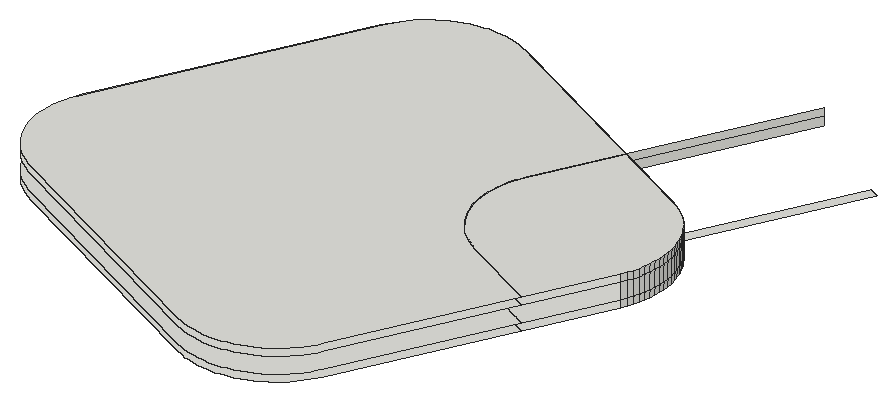
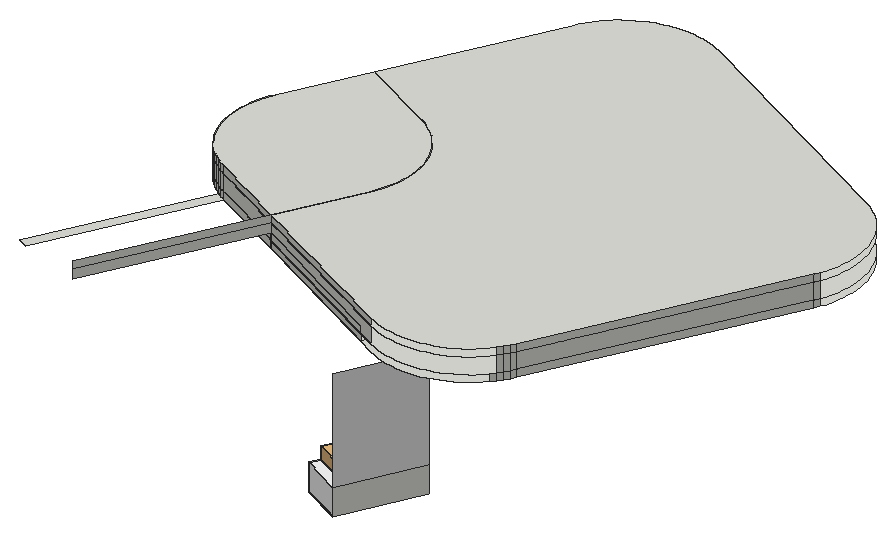
# SketchUp Ruby script. Lengths in inches.
U = 1.inch
M = Sketchup.active_model
def pt(a) = Geom::Point3d.new(a.map { |v| v * U })
def face(e, loops, mat)
  f = e.add_face(loops[0].map { |a| pt(a) })
  loops[1..].each { |l| e.add_face(l.map { |a| pt(a) }).erase! }
  f.material = f.back_material = mat if mat
  f
end
# faces: each face lists its corners as indices into pts; further lists are holes
def faces(e, pts, list, mat = nil) = list.each { |f| face(e, (f[0].is_a?(Array) ? f : [f]).map { |l| l.map { |i| pts[i] } }, mat) }
# xy, xz, yz: faces in a plane at the given z, y or x. An outline is a flat list of corners, or four numbers for a rectangle; further outlines are holes
def ring(l) = l.size == 4 ? [[l[0], l[1]], [l[2], l[1]], [l[2], l[3]], [l[0], l[3]]] : l.each_slice(2).to_a
def flat(e, list, mat, &to3) = list.each { |f| face(e, (f[0].is_a?(Array) ? f : [f]).map { |l| ring(l).map { |u, v| to3.(u, v) } }, mat) }
def xy(e, z, list, mat = nil) = flat(e, list, mat) { |x, y| [x, y, z] }
def xz(e, y, list, mat = nil) = flat(e, list, mat) { |x, z| [x, y, z] }
def yz(e, x, list, mat = nil) = flat(e, list, mat) { |y, z| [x, y, z] }
def lines(e, pts, list) = list.each { |a, b| e.add_line(pt(pts[a]), pt(pts[b])) }
# prism: a flat outline (further loops are holes) pulled along v
def prism(e, loops, v, mat = nil)
  f = face(e, loops, mat); d = Geom::Vector3d.new(v.map { |x| x * U })
  f.pushpull(f.normal.samedirection?(d) ? d.length : -d.length)
end
def box(e, o, s, mat = nil) = prism(e, [[o, [o[0] + s[0], o[1], o[2]], [o[0] + s[0], o[1] + s[1], o[2]], [o[0], o[1] + s[1], o[2]]]], [0, 0, s[2]], mat)
def at(x, y, z, deg = 0) = Geom::Transformation.translation(pt([x, y, z])) * Geom::Transformation.rotation(ORIGIN, Z_AXIS, deg.degrees)
def axes(o, x, y, z) = Geom::Transformation.new([*x, 0, *y, 0, *z, 0, *pt(o).to_a, 1])
def part(name) = M.definitions.add(name)
# library, detail: a bought-in or finely detailed component or shape, given as its bounding box
def library(name, o, s) = part(name).tap { |d| box(d.entities, o, s) }
def detail(e, o, s) = box(e.add_group.entities, o, s)
def put(e, d, t, mat = nil) = e.add_instance(d, t).tap { |i| i.material = mat if mat }
def group(e, t, mat = nil) = e.add_group.tap { |g| g.transformation = t; g.material = mat if mat }.entities
root = M.entities
M.materials.add("[Color_003]").color = [170, 170, 170]
M.materials.add("[Mirror 02]1").color = [230, 230, 230]
M.materials.add("[Plaster]").color = [253, 253, 253]
M.materials.add("[Translucent Glass Gray]14").color = [0, 0, 0]
M.materials["[Translucent Glass Gray]14"].alpha = 0.5
c1 = library("Pump dispenser pair",[-4.05,-18.11,-0.18],[3.15,7.24,8.23])
c2 = library("グループ\#54",[0,0,0],[6.36,0.94,9.53])
c3 = library("グループ\#83",[0,0.04,0],[11.77,11.73,3.9375])
c4 = part("Untitled1")
g1 = group(c4.entities,at(743.43,-253.09,0,-180))
xy(g1,0,[[0,0,554.6,297.75]],"[Plaster]")
xy(g1,29.71,[[41.91,287.06,269.97,291.99],[269.97,287.06,498.03,291.99]])
xy(g1,29.71,[[41.91,170.9375,498.03,287.06],[41.91,291.99,498.03,297.75]],"[Plaster]")
xy(g1,101.91,[[120.41,291.99,133.72,291.99,133.72,305.17,218.84,305.17,218.84,291.99,232.79,291.99,232.79,311.8,120.41,311.8],[305.71,291.99,312.55,291.99,312.55,305.42,407.55,305.42,407.55,291.99,418.08,291.99,418.08,312.8,305.71,312.8]],"[Translucent Glass Gray]14")
xy(g1,110.16,[[120.41,291.99,120.41,311.8,232.79,311.8,232.79,291.99,218.84,291.99,218.84,305.17,133.72,305.17,133.72,291.99],[305.71,291.99,305.71,312.8,418.08,312.8,418.08,291.99,407.55,291.99,407.55,305.42,312.55,305.42,312.55,291.99]],"[Translucent Glass Gray]14")
xy(g1,152.15,[[41.91,287.06,269.97,291.99],[269.97,287.06,498.03,291.99]])
xy(g1,152.15,[[41.91,170.9375,498.03,287.06],[41.91,291.99,498.03,297.75]],"[Plaster]")
xy(g1,175.18,[[0,0,554.6,297.75]],"[Plaster]")
xz(g1,0,[[0,0,554.6,175.18]])
xz(g1,0,[[0,175.18,554.6,861.94]],"[Mirror 02]1")
xz(g1,170.9375,[[41.91,29.71,498.03,152.15]],"[Plaster]")
xz(g1,287.06,[[41.91,29.71,269.97,152.15],[269.97,29.71,498.03,152.15]],"[Translucent Glass Gray]14")
xz(g1,291.99,[[[41.91,29.71,269.97,152.15],[218.84,101.91,232.79,110.16],[120.41,101.91,133.72,110.16]],[[269.97,29.71,498.03,152.15],[407.55,101.91,418.08,110.16],[305.71,101.91,312.55,110.16]]],"[Translucent Glass Gray]14")
xz(g1,297.75,[[[0,0,554.6,175.18],[41.91,29.71,498.03,152.15]]],"[Plaster]")
xz(g1,305.17,[[133.72,101.91,218.84,110.16]],"[Translucent Glass Gray]14")
xz(g1,305.42,[[312.55,101.91,407.55,110.16]],"[Translucent Glass Gray]14")
xz(g1,311.8,[[120.41,101.91,232.79,110.16]],"[Translucent Glass Gray]14")
xz(g1,312.8,[[305.71,101.91,418.08,110.16]],"[Translucent Glass Gray]14")
yz(g1,0,[[0,0,297.75,175.18]],"[Plaster]")
yz(g1,41.91,[[170.9375,29.71,287.06,152.15],[291.99,29.71,297.75,152.15]],"[Plaster]")
yz(g1,41.91,[[287.06,29.71,291.99,152.15]],"[Translucent Glass Gray]14")
yz(g1,120.41,[[291.99,101.91,311.8,110.16]],"[Translucent Glass Gray]14")
yz(g1,133.72,[[291.99,101.91,305.17,110.16]],"[Translucent Glass Gray]14")
yz(g1,218.84,[[291.99,101.91,305.17,110.16]],"[Translucent Glass Gray]14")
yz(g1,232.79,[[291.99,101.91,311.8,110.16]],"[Translucent Glass Gray]14")
yz(g1,269.97,[[287.06,29.71,291.99,152.15]],"[Translucent Glass Gray]14")
yz(g1,305.71,[[291.99,101.91,312.8,110.16]],"[Translucent Glass Gray]14")
yz(g1,312.55,[[291.99,101.91,305.42,110.16]],"[Translucent Glass Gray]14")
yz(g1,407.55,[[291.99,101.91,305.42,110.16]],"[Translucent Glass Gray]14")
yz(g1,418.08,[[291.99,101.91,312.8,110.16]],"[Translucent Glass Gray]14")
yz(g1,498.03,[[287.06,29.71,291.99,152.15]])
yz(g1,498.03,[[170.9375,29.71,287.06,152.15],[291.99,29.71,297.75,152.15]],"[Plaster]")
yz(g1,554.6,[[0,0,297.75,175.18]])
put(g1,c1,axes([334.9,116.79,177.8],[0,14.82,0],[-11.7078,0,0],[0,0,14.82]))
g2 = group(g1,at(68.38,2.16,176.47))
put(g2,c2,axes([147.62,131.72,21.69],[0,-20.70307,0],[29.98633,0,0],[0,0,20.70307]),"[Color_003]")
put(g2,c3,axes([-1.1,49.75,0],[0,20.70307,0],[29.98633,0,0],[0,0,20.70307]))
xy(root,412.84,[[[714.28,690.62,711.93,690.68,709.58,690.9,707.25,691.27,704.96,691.79,702.7,692.46,700.49,693.28,698.34,694.23,596.96,743.46,594.88,744.56,592.87,745.79,590.95,747.15,589.12,748.63,587.39,750.23,585.77,751.94,584.26,753.75,582.88,755.66,581.625,757.65,580.5,759.72,579.51,761.86,578.67,764.0625,577.97,766.3125,577.43,768.6,577.03,770.92,576.78,773.27,576.69,775.62,576.75,777.98,576.97,780.32,577.34,782.65,577.86,784.95,578.53,787.2,579.35,789.41,580.31,791.57,627.47,888.7,628.57,890.78,629.8,892.79,631.16,894.71,632.64,896.54,634.24,898.27,635.95,899.89,637.76,901.4,639.67,902.78,641.66,904.04,643.73,905.16,645.875,906.15,648.07,906.99,650.32,907.6875,652.61,908.24,654.9375,908.63,657.28,908.88,659.63,908.97,661.99,908.91,664.33,908.69,666.66,908.32,668.96,907.8,671.22,907.13,673.43,906.3125,675.58,905.36,682.44,902.02,666.72,869.64,671.22,867.45,686.94,899.84,744.57,871.86,728.84,839.47,727.88,837.32,727.06,835.11,726.39,832.85,725.875,830.56,725.5,828.23,725.29,825.88,725.23,823.53,725.32,821.17,725.5625,818.83,725.96,816.51,726.51,814.22,727.21,811.97,728.05,809.77,729.03,807.63,730.16,805.56,731.41,803.57,732.8,801.66,734.3,799.85,735.92,798.14,737.65,796.54,739.48,795.05,741.41,793.69,743.42,792.46,745.5,791.36,777.88,775.64,746.44,710.89,745.35,708.81,744.12,706.8,742.75,704.88,741.27,703.05,739.67,701.32,737.96,699.7,736.15,698.19,734.24,696.81,732.25,695.55,730.18,694.43,728.04,693.44,725.84,692.6,723.59,691.9,721.3,691.35,718.98,690.96,716.63,690.71],[616.59,773.95,663.75,871.08,659.85,872.97,612.69,775.84],[703.25,736.11,705.125,736.17,706.96,736.32,708.74,736.59,710.47,736.95,712.14,737.42,713.73,737.98,715.25,738.65,716.69,739.4,718.04,740.25,719.29,741.1875,720.45,742.2,721.5,743.3,722.43,744.47,723.26,745.72,723.97,747.02,729.79,759,728.6875,756.92,727.46,754.91,726.1,752.99,724.61,751.16,723.01,749.43,721.3,747.81,719.49,746.3,717.58,744.92,716.26,744.08,716.04,743.89,714.96,743.09,713.8,742.36,712.5625,741.7,711.25,741.13,709.88,740.65,708.44,740.24,706.96,739.93,706.02,739.79,704.64,739.46,702.32,739.06,699.98,738.82,697.62,738.73,695.27,738.79,692.92,739.01,690.59,739.375,688.3,739.9,686.04,740.57,683.83,741.38,681.68,742.34,685.99,740.25,687.85,739.4,689.74,738.64,691.66,737.98,693.59,737.42,695.54,736.95,697.49,736.59,699.43,736.32,701.35,736.17]],[616.59,773.95,612.69,775.84,659.85,872.97,663.75,871.08],[[777.88,775.64,745.5,791.36,743.42,792.46,741.41,793.69,739.48,795.05,737.65,796.54,735.92,798.14,734.3,799.85,732.8,801.66,731.41,803.57,730.16,805.56,729.03,807.63,728.05,809.77,727.21,811.97,726.51,814.22,725.96,816.51,725.5625,818.83,725.32,821.17,725.23,823.53,725.29,825.88,725.5,828.23,725.875,830.56,726.39,832.85,727.06,835.11,727.88,837.32,728.84,839.47,744.57,871.86,744.58,871.85,744.84,871.72,776.95,856.13,779.03,855.03,781.04,853.8,782.97,852.44,784.8,850.96,786.52,849.36,788.15,847.65,789.65,845.84,791.03,843.93,792.29,841.9375,793.41,839.87,794.4,837.73,795.24,835.53,795.94,833.28,796.49,830.99,796.89,828.67,797.13,826.32,797.22,823.97,797.16,821.61,796.94,819.27,796.58,816.94,796.05,814.64,795.38,812.38,794.57,810.18,793.61,808.02],[765.125,821.85,767.29,826.32,762.79,828.5,760.625,824.04]],[765.125,821.85,760.625,824.04,762.79,828.5,767.29,826.32],[780.85,854.24,776.95,856.13,808.39,920.88,812.29,918.98],
  [671.22,867.45,686.94,899.84,682.44,902.02,666.72,869.64]])
xy(root,415.76,[[714.28,690.62,711.93,690.68,709.58,690.9,707.25,691.27,704.96,691.79,702.7,692.46,700.49,693.28,698.34,694.23,596.96,743.46,594.88,744.56,592.87,745.79,590.95,747.15,589.12,748.63,587.39,750.23,585.77,751.94,584.26,753.75,582.88,755.66,581.625,757.65,580.5,759.72,579.51,761.86,578.67,764.0625,577.97,766.3125,577.43,768.6,577.03,770.92,576.78,773.27,576.69,775.62,576.75,777.98,576.97,780.32,577.34,782.65,577.86,784.95,578.53,787.2,579.35,789.41,580.31,791.57,627.47,888.7,628.57,890.78,629.8,892.79,631.16,894.71,632.64,896.54,634.24,898.27,635.95,899.89,637.76,901.4,639.67,902.78,641.66,904.04,643.73,905.16,645.875,906.15,648.07,906.99,650.32,907.6875,652.61,908.24,654.9375,908.63,657.28,908.88,659.63,908.97,661.99,908.91,664.33,908.69,666.66,908.32,668.96,907.8,671.22,907.13,673.43,906.3125,675.58,905.36,682.44,902.02,744.57,871.86,728.84,839.47,727.88,837.32,727.06,835.11,726.39,832.85,725.875,830.56,725.5,828.23,725.29,825.88,725.23,823.53,725.32,821.17,725.5625,818.83,725.96,816.51,726.51,814.22,727.21,811.97,728.05,809.77,729.03,807.63,730.16,805.56,731.41,803.57,732.8,801.66,734.3,799.85,735.92,798.14,737.65,796.54,739.48,795.05,741.41,793.69,743.42,792.46,745.5,791.36,777.88,775.64,746.44,710.89,745.35,708.81,744.12,706.8,742.75,704.88,741.27,703.05,739.67,701.32,737.96,699.7,736.15,698.19,734.24,696.81,732.25,695.55,730.18,694.43,728.04,693.44,725.84,692.6,723.59,691.9,721.3,691.35,718.98,690.96,716.63,690.71],[777.88,775.64,745.5,791.36,743.42,792.46,741.41,793.69,739.48,795.05,737.65,796.54,735.92,798.14,734.3,799.85,732.8,801.66,731.41,803.57,730.16,805.56,729.03,807.63,728.05,809.77,727.21,811.97,726.51,814.22,725.96,816.51,725.5625,818.83,725.32,821.17,725.23,823.53,725.29,825.88,725.5,828.23,725.875,830.56,726.39,832.85,727.06,835.11,727.88,837.32,728.84,839.47,744.57,871.86,744.84,871.72,776.95,856.13,779.03,855.03,781.04,853.8,782.97,852.44,784.8,850.96,786.52,849.36,788.15,847.65,789.65,845.84,791.03,843.93,792.29,841.9375,793.41,839.87,794.4,837.73,795.24,835.53,795.94,833.28,796.49,830.99,796.89,828.67,797.13,826.32,797.22,823.97,797.16,821.61,796.94,819.27,796.58,816.94,796.05,814.64,795.38,812.38,794.57,810.18,793.61,808.02]])
xy(root,422.51,[[714.28,690.62,711.93,690.68,709.58,690.9,707.25,691.27,704.96,691.79,702.7,692.46,700.49,693.28,698.34,694.23,596.96,743.46,594.88,744.56,592.87,745.79,590.95,747.15,589.12,748.63,587.39,750.23,585.77,751.94,584.26,753.75,582.88,755.66,581.625,757.65,580.5,759.72,579.51,761.86,578.67,764.0625,577.97,766.3125,577.43,768.6,577.03,770.92,576.78,773.27,576.69,775.62,576.75,777.98,576.97,780.32,577.34,782.65,577.86,784.95,578.53,787.2,579.35,789.41,580.31,791.57,627.47,888.7,628.57,890.78,629.8,892.79,631.16,894.71,632.64,896.54,634.24,898.27,635.95,899.89,637.76,901.4,639.67,902.78,641.66,904.04,643.73,905.16,645.875,906.15,648.07,906.99,650.32,907.6875,652.61,908.24,654.9375,908.63,657.28,908.88,659.63,908.97,661.99,908.91,664.33,908.69,666.66,908.32,668.96,907.8,671.22,907.13,673.43,906.3125,675.58,905.36,744.57,871.86,728.84,839.47,727.88,837.32,727.06,835.11,726.39,832.85,725.875,830.56,725.5,828.23,725.29,825.88,725.23,823.53,725.32,821.17,725.5625,818.83,725.96,816.51,726.51,814.22,727.21,811.97,728.05,809.77,729.03,807.63,730.16,805.56,731.41,803.57,732.8,801.66,734.3,799.85,735.92,798.14,737.65,796.54,739.48,795.05,741.41,793.69,743.42,792.46,745.5,791.36,777.88,775.64,746.44,710.89,745.35,708.81,744.12,706.8,742.75,704.88,741.27,703.05,739.67,701.32,737.96,699.7,736.15,698.19,734.24,696.81,732.25,695.55,730.18,694.43,728.04,693.44,725.84,692.6,723.59,691.9,721.3,691.35,718.98,690.96,716.63,690.71],[777.88,775.64,745.5,791.36,743.42,792.46,741.41,793.69,739.48,795.05,737.65,796.54,735.92,798.14,734.3,799.85,732.8,801.66,731.41,803.57,730.16,805.56,729.03,807.63,728.05,809.77,727.21,811.97,726.51,814.22,725.96,816.51,725.5625,818.83,725.32,821.17,725.23,823.53,725.29,825.88,725.5,828.23,725.875,830.56,726.39,832.85,727.06,835.11,727.88,837.32,728.84,839.47,744.57,871.86,776.95,856.13,779.03,855.03,781.04,853.8,782.97,852.44,784.8,850.96,786.52,849.36,788.15,847.65,789.65,845.84,791.03,843.93,792.29,841.9375,793.41,839.87,794.4,837.73,795.24,835.53,795.94,833.28,796.49,830.99,796.89,828.67,797.13,826.32,797.22,823.97,797.16,821.61,796.94,819.27,796.58,816.94,796.05,814.64,795.38,812.38,794.57,810.18,793.61,808.02]])
xy(root,425.53,[[714.28,690.62,716.63,690.71,718.98,690.96,721.3,691.35,723.59,691.9,725.84,692.6,728.04,693.44,730.18,694.43,732.25,695.55,734.24,696.81,736.15,698.19,737.96,699.7,739.67,701.32,741.27,703.05,742.75,704.88,744.12,706.8,745.35,708.81,746.44,710.89,777.88,775.64,745.5,791.36,743.42,792.46,741.41,793.69,739.48,795.05,737.65,796.54,735.92,798.14,734.3,799.85,732.8,801.66,731.41,803.57,730.16,805.56,729.03,807.63,728.05,809.77,727.21,811.97,726.51,814.22,725.96,816.51,725.5625,818.83,725.32,821.17,725.23,823.53,725.29,825.88,725.5,828.23,725.875,830.56,726.39,832.85,727.06,835.11,727.88,837.32,728.84,839.47,744.57,871.86,675.58,905.36,673.43,906.3125,671.22,907.13,668.96,907.8,666.66,908.32,664.33,908.69,661.99,908.91,659.63,908.97,657.28,908.88,654.9375,908.63,652.61,908.24,650.32,907.6875,648.07,906.99,645.875,906.15,643.73,905.16,641.66,904.04,639.67,902.78,637.76,901.4,635.95,899.89,634.24,898.27,632.64,896.54,631.16,894.71,629.8,892.79,628.57,890.78,627.47,888.7,580.31,791.57,579.35,789.41,578.53,787.2,577.86,784.95,577.34,782.65,576.97,780.32,576.75,777.98,576.69,775.62,576.78,773.27,577.03,770.92,577.43,768.6,577.97,766.3125,578.67,764.0625,579.51,761.86,580.5,759.72,581.625,757.65,582.88,755.66,584.26,753.75,585.77,751.94,587.39,750.23,589.12,748.63,590.95,747.15,592.87,745.79,594.88,744.56,596.96,743.46,698.34,694.23,700.49,693.28,702.7,692.46,704.96,691.79,707.25,691.27,709.58,690.9,711.93,690.68],[777.88,775.64,793.61,808.02,794.57,810.18,795.38,812.38,796.05,814.64,796.58,816.94,796.94,819.27,797.16,821.61,797.22,823.97,797.13,826.32,796.89,828.67,796.49,830.99,795.94,833.28,795.24,835.53,794.4,837.73,793.41,839.87,792.29,841.9375,791.03,843.93,789.65,845.84,788.15,847.65,786.52,849.36,784.8,850.96,782.97,852.44,781.04,853.8,779.03,855.03,776.95,856.13,744.57,871.86,728.84,839.47,727.88,837.32,727.06,835.11,726.39,832.85,725.875,830.56,725.5,828.23,725.29,825.88,725.23,823.53,725.32,821.17,725.5625,818.83,725.96,816.51,726.51,814.22,727.21,811.97,728.05,809.77,729.03,807.63,730.16,805.56,731.41,803.57,732.8,801.66,734.3,799.85,735.92,798.14,737.65,796.54,739.48,795.05,741.41,793.69,743.42,792.46,745.5,791.36]])
p = [[580.31,791.57,415.76],[580.31,791.57,412.84],[579.35,789.41,412.84],[579.35,789.41,415.76],[743.42,792.46,415.76],[743.42,792.46,412.84],
  [745.5,791.36,412.84],[745.5,791.36,415.76],[627.47,888.7,412.84],[627.47,888.7,415.76],[741.41,793.69,415.76],[741.41,793.69,412.84],
  [739.48,795.05,415.76],[739.48,795.05,412.84],[737.65,796.54,415.76],[737.65,796.54,412.84],[735.92,798.14,415.76],[735.92,798.14,412.84],
  [734.3,799.85,415.76],[734.3,799.85,412.84],[732.8,801.66,415.76],[732.8,801.66,412.84],[731.41,803.57,415.76],[731.41,803.57,412.84],
  [730.16,805.56,415.76],[730.16,805.56,412.84],[729.03,807.63,415.76],[729.03,807.63,412.84],[728.05,809.77,415.76],[728.05,809.77,412.84],
  [794.57,810.18,412.84],[794.57,810.18,415.76],[793.61,808.02,415.76],[793.61,808.02,412.84],[727.21,811.97,415.76],[727.21,811.97,412.84],
  [795.38,812.38,412.84],[795.38,812.38,415.76],[726.51,814.22,415.76],[726.51,814.22,412.84],[796.05,814.64,412.84],[796.05,814.64,415.76],
  [725.96,816.51,415.76],[725.96,816.51,412.84],[796.58,816.94,412.84],[796.58,816.94,415.76],[725.5625,818.83,415.76],[725.5625,818.83,412.84],
  [796.94,819.27,412.84],[796.94,819.27,415.76],[725.32,821.17,415.76],[725.32,821.17,412.84],[797.16,821.61,412.84],[797.16,821.61,415.76],
  [725.23,823.53,415.76],[725.23,823.53,412.84],[797.22,823.97,412.84],[797.22,823.97,415.76],[725.29,825.88,415.76],[725.29,825.88,412.84],
  [797.13,826.32,412.84],[797.13,826.32,415.76],[725.5,828.23,415.76],[725.5,828.23,412.84],[796.89,828.67,412.84],[796.89,828.67,415.76],
  [725.875,830.56,415.76],[725.875,830.56,412.84],[796.49,830.99,412.84],[796.49,830.99,415.76],[726.39,832.85,415.76],[726.39,832.85,412.84],
  [795.94,833.28,412.84],[795.94,833.28,415.76],[727.06,835.11,415.76],[727.06,835.11,412.84],[795.24,835.53,412.84],[795.24,835.53,415.76],
  [727.88,837.32,415.76],[727.88,837.32,412.84],[794.4,837.73,412.84],[794.4,837.73,415.76],[728.84,839.47,415.76],[728.84,839.47,412.84],
  [793.41,839.87,412.84],[793.41,839.87,415.76],[744.57,871.86,415.76],[744.57,871.86,412.84],[792.29,841.9375,412.84],[792.29,841.9375,415.76],
  [791.03,843.93,412.84],[791.03,843.93,415.76],[789.65,845.84,412.84],[789.65,845.84,415.76],[788.15,847.65,412.84],[788.15,847.65,415.76],
  [786.52,849.36,412.84],[786.52,849.36,415.76],[784.8,850.96,412.84],[784.8,850.96,415.76],[782.97,852.44,412.84],[782.97,852.44,415.76],
  [781.04,853.8,412.84],[781.04,853.8,415.76],[779.03,855.03,412.84],[779.03,855.03,415.76],[776.95,856.13,412.84],[776.95,856.13,415.76],
  [744.84,871.72,412.84],[744.84,871.72,415.76],[744.58,871.85,412.84],[682.44,902.02,415.76],[686.94,899.84,412.84],[682.44,902.02,412.84],
  [628.57,890.78,415.76],[628.57,890.78,412.84],[629.8,892.79,415.76],[629.8,892.79,412.84],[631.16,894.71,415.76],[631.16,894.71,412.84],
  [632.64,896.54,415.76],[632.64,896.54,412.84],[579.35,789.41,422.51],[580.31,791.57,422.51],[745.5,791.36,422.51],[743.42,792.46,422.51],
  [627.47,888.7,422.51],[741.41,793.69,422.51],[739.48,795.05,422.51],[737.65,796.54,422.51],[735.92,798.14,422.51],[734.3,799.85,422.51],
  [732.8,801.66,422.51],[731.41,803.57,422.51],[730.16,805.56,422.51],[729.03,807.63,422.51],[728.05,809.77,422.51],[794.57,810.18,422.51],
  [793.61,808.02,422.51],[727.21,811.97,422.51],[795.38,812.38,422.51],[726.51,814.22,422.51],[796.05,814.64,422.51],[725.96,816.51,422.51],
  [796.58,816.94,422.51],[725.5625,818.83,422.51],[796.94,819.27,422.51],[725.32,821.17,422.51],[797.16,821.61,422.51],[725.23,823.53,422.51],
  [797.22,823.97,422.51],[725.29,825.88,422.51],[797.13,826.32,422.51],[725.5,828.23,422.51],[796.89,828.67,422.51],[725.875,830.56,422.51],
  [796.49,830.99,422.51],[726.39,832.85,422.51],[795.94,833.28,422.51],[727.06,835.11,422.51],[795.24,835.53,422.51],[727.88,837.32,422.51],
  [794.4,837.73,422.51],[728.84,839.47,422.51],[793.41,839.87,422.51],[776,936.6,422.51],[776,936.6,418.84],[744.57,871.86,418.84],
  [744.57,871.86,422.51],[792.29,841.9375,422.51],[791.03,843.93,422.51],[789.65,845.84,422.51],[788.15,847.65,422.51],[786.52,849.36,422.51],
  [784.8,850.96,422.51],[782.97,852.44,422.51],[781.04,853.8,422.51],[779.03,855.03,422.51],[776.95,856.13,422.51],[682.44,902.02,418.84],
  [675.58,905.36,415.76],[675.58,905.36,422.51],[628.57,890.78,422.51],[629.8,892.79,422.51],[631.16,894.71,422.51],[579.35,789.41,425.53],
  [580.31,791.57,425.53],[745.5,791.36,425.53],[743.42,792.46,425.53],[627.47,888.7,425.53],[741.41,793.69,425.53],[739.48,795.05,425.53],
  [737.65,796.54,425.53],[735.92,798.14,425.53],[734.3,799.85,425.53],[732.8,801.66,425.53],[731.41,803.57,425.53],[730.16,805.56,425.53],
  [729.03,807.63,425.53],[728.05,809.77,425.53],[794.57,810.18,425.53],[793.61,808.02,425.53],[727.21,811.97,425.53],[795.38,812.38,425.53],
  [726.51,814.22,425.53],[796.05,814.64,425.53],[725.96,816.51,425.53],[796.58,816.94,425.53],[725.5625,818.83,425.53],[796.94,819.27,425.53],
  [725.32,821.17,425.53],[797.16,821.61,425.53],[725.23,823.53,425.53],[797.22,823.97,425.53],[725.29,825.88,425.53],[797.13,826.32,425.53],
  [725.5,828.23,425.53],[796.89,828.67,425.53],[725.875,830.56,425.53],[796.49,830.99,425.53],[726.39,832.85,425.53],[795.94,833.28,425.53],
  [727.06,835.11,425.53],[795.24,835.53,425.53],[727.88,837.32,425.53],[794.4,837.73,425.53],[728.84,839.47,425.53],[793.41,839.87,425.53],
  [744.57,871.86,425.53],[776,936.6,425.53],[792.29,841.9375,425.53],[791.03,843.93,425.53],[789.65,845.84,425.53],[788.15,847.65,425.53],
  [786.52,849.36,425.53],[784.8,850.96,425.53],[782.97,852.44,425.53],[781.04,853.8,425.53],[779.03,855.03,425.53],[776.95,856.13,425.53],
  [675.58,905.36,425.53],[628.57,890.78,425.53],[629.8,892.79,425.53],[631.16,894.71,425.53]]
faces(root,p,[[0,1,2,3],[4,5,6,7],[8,1,0,9],[10,11,5,4],[12,13,11,10],[14,15,13,12],[16,17,15,14],[18,19,17,16],
  [20,21,19,18],[22,23,21,20],[24,25,23,22],[26,27,25,24],[28,29,27,26],[30,31,32,33],[34,35,29,28],[36,37,31,30],
  [38,39,35,34],[40,41,37,36],[42,43,39,38],[44,45,41,40],[46,47,43,42],[48,49,45,44],[50,51,47,46],[52,53,49,48],
  [54,55,51,50],[56,57,53,52],[58,59,55,54],[60,61,57,56],[62,63,59,58],[64,65,61,60],[66,67,63,62],[68,69,65,64],
  [70,71,67,66],[72,73,69,68],[74,75,71,70],[76,77,73,72],[78,79,75,74],[80,81,77,76],[82,83,79,78],[84,85,81,80],
  [82,86,87,83],[88,89,85,84],[90,91,89,88],[92,93,91,90],[94,95,93,92],[96,97,95,94],[98,99,97,96],[100,101,99,98],
  [102,103,101,100],[104,105,103,102],[106,107,105,104],[106,108,109,107],[110,87,86,109,108],[111,86,87,112,113],[114,115,8,9],[116,117,115,114],
  [118,119,117,116],[120,121,119,118],[0,3,122,123],[4,7,124,125],[9,0,123,126],[10,4,125,127],[12,10,127,128],[14,12,128,129],
  [16,14,129,130],[18,16,130,131],[20,18,131,132],[22,20,132,133],[24,22,133,134],[26,24,134,135],[28,26,135,136],[32,31,137,138],
  [34,28,136,139],[31,37,140,137],[38,34,139,141],[37,41,142,140],[42,38,141,143],[41,45,144,142],[46,42,143,145],[45,49,146,144],
  [50,46,145,147],[49,53,148,146],[54,50,147,149],[53,57,150,148],[58,54,149,151],[57,61,152,150],[62,58,151,153],[61,65,154,152],
  [66,62,153,155],[65,69,156,154],[70,66,155,157],[69,73,158,156],[74,70,157,159],[73,77,160,158],[78,74,159,161],[77,81,162,160],
  [82,78,161,163],[81,85,164,162],[165,166,167,86,82,163,168],[85,89,169,164],[89,91,170,169],[91,93,171,170],[93,95,172,171],[95,97,173,172],
  [97,99,174,173],[99,101,175,174],[101,103,176,175],[103,105,177,176],[105,107,178,177],[109,86,167,179,111,180,181,168,178,107],[111,86,167,179],[114,9,126,182],
  [116,114,182,183],[118,116,183,184],[123,122,185,186],[125,124,187,188],[126,123,186,189],[127,125,188,190],[128,127,190,191],[129,128,191,192],
  [130,129,192,193],[131,130,193,194],[132,131,194,195],[133,132,195,196],[134,133,196,197],[135,134,197,198],[136,135,198,199],[138,137,200,201],
  [139,136,199,202],[137,140,203,200],[141,139,202,204],[140,142,205,203],[143,141,204,206],[142,144,207,205],[145,143,206,208],[144,146,209,207],
  [147,145,208,210],[146,148,211,209],[149,147,210,212],[148,150,213,211],[151,149,212,214],[150,152,215,213],[153,151,214,216],[152,154,217,215],
  [155,153,216,218],[154,156,219,217],[157,155,218,220],[156,158,221,219],[159,157,220,222],[158,160,223,221],[161,159,222,224],[160,162,225,223],
  [163,161,224,226],[162,164,227,225],[165,168,163,226,228,229],[164,169,230,227],[169,170,231,230],[170,171,232,231],[171,172,233,232],[172,173,234,233],
  [173,174,235,234],[174,175,236,235],[175,176,237,236],[176,177,238,237],[177,178,239,238],[178,168,181,240,228,239],[182,126,189,241],[183,182,241,242],
  [184,183,242,243]])
put(root,c4,axes([655.8,871.91,346.15],[0.0273,0.05622,0],[-0.05622,0.0273,0],[0,0,0.0625]))
